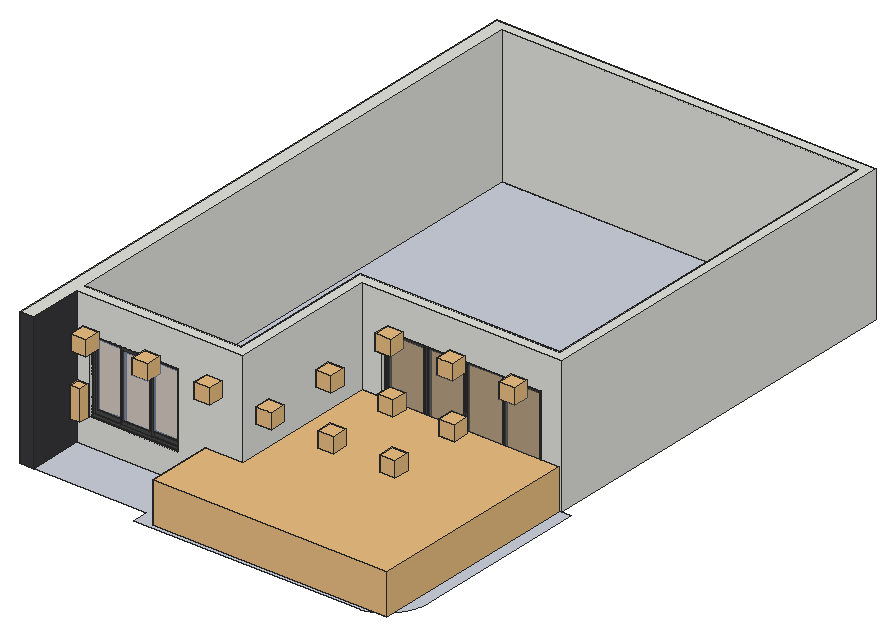
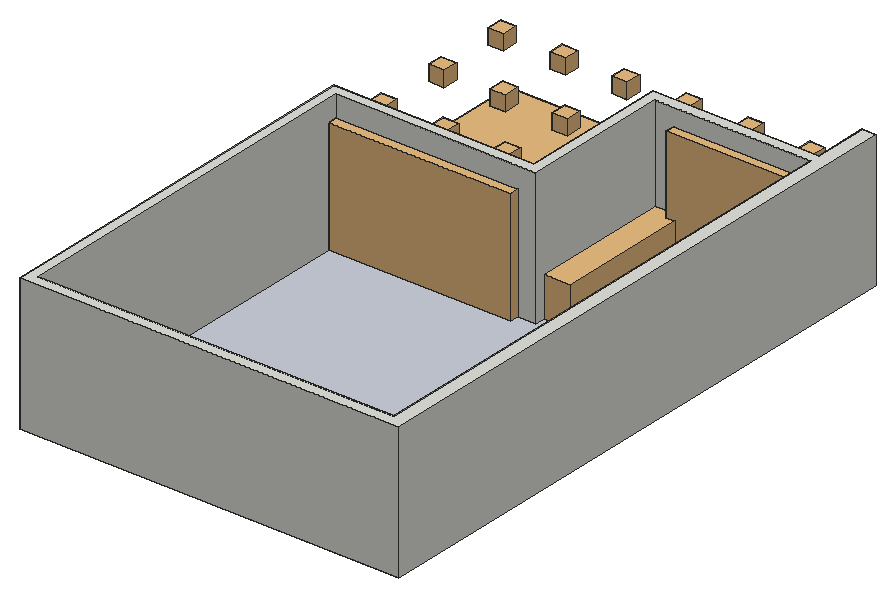
# SketchUp Ruby script. Lengths in inches.
U = 1.inch
M = Sketchup.active_model
def pt(a) = Geom::Point3d.new(a.map { |v| v * U })
def face(e, loops, mat)
  f = e.add_face(loops[0].map { |a| pt(a) })
  loops[1..].each { |l| e.add_face(l.map { |a| pt(a) }).erase! }
  f.material = f.back_material = mat if mat
  f
end
# faces: each face lists its corners as indices into pts; further lists are holes
def faces(e, pts, list, mat = nil) = list.each { |f| face(e, (f[0].is_a?(Array) ? f : [f]).map { |l| l.map { |i| pts[i] } }, mat) }
# xy, xz, yz: faces in a plane at the given z, y or x. An outline is a flat list of corners, or four numbers for a rectangle; further outlines are holes
def ring(l) = l.size == 4 ? [[l[0], l[1]], [l[2], l[1]], [l[2], l[3]], [l[0], l[3]]] : l.each_slice(2).to_a
def flat(e, list, mat, &to3) = list.each { |f| face(e, (f[0].is_a?(Array) ? f : [f]).map { |l| ring(l).map { |u, v| to3.(u, v) } }, mat) }
def xy(e, z, list, mat = nil) = flat(e, list, mat) { |x, y| [x, y, z] }
def xz(e, y, list, mat = nil) = flat(e, list, mat) { |x, z| [x, y, z] }
def yz(e, x, list, mat = nil) = flat(e, list, mat) { |y, z| [x, y, z] }
def lines(e, pts, list) = list.each { |a, b| e.add_line(pt(pts[a]), pt(pts[b])) }
# prism: a flat outline (further loops are holes) pulled along v
def prism(e, loops, v, mat = nil)
  f = face(e, loops, mat); d = Geom::Vector3d.new(v.map { |x| x * U })
  f.pushpull(f.normal.samedirection?(d) ? d.length : -d.length)
end
def box(e, o, s, mat = nil) = prism(e, [[o, [o[0] + s[0], o[1], o[2]], [o[0] + s[0], o[1] + s[1], o[2]], [o[0], o[1] + s[1], o[2]]]], [0, 0, s[2]], mat)
def at(x, y, z, deg = 0) = Geom::Transformation.translation(pt([x, y, z])) * Geom::Transformation.rotation(ORIGIN, Z_AXIS, deg.degrees)
def axes(o, x, y, z) = Geom::Transformation.new([*x, 0, *y, 0, *z, 0, *pt(o).to_a, 1])
def part(name) = M.definitions.add(name)
# library, detail: a bought-in or finely detailed component or shape, given as its bounding box
def library(name, o, s) = part(name).tap { |d| box(d.entities, o, s) }
def detail(e, o, s) = box(e.add_group.entities, o, s)
def put(e, d, t, mat = nil) = e.add_instance(d, t).tap { |i| i.material = mat if mat }
def group(e, t, mat = nil) = e.add_group.tap { |g| g.transformation = t; g.material = mat if mat }.entities
root = M.entities
M.materials.add("1432 AP 8245 TAR ROAD").color = [57, 57, 60]
M.materials.add("[Marble Carrara Floor Tile]").color = [204, 208, 219]
M.materials.add("[Steel Brushed Stainless]").color = [71, 71, 71]
M.materials.add("[Steel Brushed Stainless]1").color = [76, 76, 76]
M.materials.add("[Translucent Glass Blue]").color = [188, 212, 255]
M.materials["[Translucent Glass Blue]"].alpha = 0.5
M.materials.add("[Translucent Glass Gray]").color = [128, 128, 128]
M.materials["[Translucent Glass Gray]"].alpha = 0.5
c1 = part("Group\#13")
box(c1.entities,[0,0,0],[1.97,3.9375,10.02])
c2 = part("Group\#9")
box(c2.entities,[0,2.36,0.1],[1.97,1.58,9.67])
c3 = part("Group\#10")
xz(c3.entities,0,[[0,0,33.34,51.88]])
c4 = part("Group\#11")
xy(c4.entities,0.1,[[0,2.36,1.97,3.9375]])
xy(c4.entities,4.64,[[0.39,2.36,1.57,2.95]])
xy(c4.entities,5.23,[[0.39,2.36,1.57,2.95]])
xy(c4.entities,9.77,[[0,2.36,1.97,3.9375]])
xz(c4.entities,2.36,[[[0,0.1,1.97,9.77],[0.39,4.64,1.57,5.23]]])
xz(c4.entities,2.95,[[0.39,4.64,1.57,5.23]])
xz(c4.entities,3.9375,[[0,0.1,1.97,9.77]])
yz(c4.entities,0,[[2.36,0.1,3.9375,9.77]])
yz(c4.entities,0.39,[[2.36,4.64,2.95,5.23]])
yz(c4.entities,1.57,[[2.36,4.64,2.95,5.23]])
yz(c4.entities,1.97,[[2.36,0.1,3.9375,9.77]])
c5 = part("slide door")
p = [[0,0,0],[118.11,0,0],[0,0,80.71],[0,-3.9375,80.71],[93.24,-3.9375,80.71]]
lines(c5.entities,p,[[0,1],[2,0],[3,4]])
put(c5.entities,c1,axes([116.56,-3.9375,0],[0.78947,0,0],[0,1,0],[0,0,8.05818]))
put(c5.entities,c1,axes([0,-3.9375,0],[0.78947,0,0],[0,1,0],[0,0,8.05818]))
put(c5.entities,c1,axes([1.55,-3.9375,80.71],[0,0,-1],[0,1,0],[11.48213,0,0]))
g1 = group(c5.entities,at(1.55,-3.9375,1.97))
box(g1,[0,0,-1.97],[115,3.9375,0.79])
put(c5.entities,c2,axes([1.55,-5.91,0],[0.78947,0,0],[0,1,0],[0,0,8.05818]))
put(c5.entities,c2,axes([28.75,-5.91,0],[0.78947,0,0],[0,1,0],[0,0,8.05818]))
put(c5.entities,c2,axes([2.85,-5.91,2.76],[0,0,-1],[0,1,0],[2.65072,0,0]))
put(c5.entities,c2,axes([2.85,-5.91,78.74],[0,0,-1],[0,1,0],[2.65072,0,0]))
put(c5.entities,c3,axes([3.11,-2.76,2.76],[0.76906,0,0],[0,1,0],[0,0,1.42673]),"[Translucent Glass Gray]")
put(c5.entities,c2,axes([89.1,-5.91,78.74],[0,0,-1],[0,1,0],[2.65072,0,0]))
put(c5.entities,c3,axes([89.36,-2.76,2.76],[0.76906,0,0],[0,1,0],[0,0,1.42673]),"[Translucent Glass Gray]")
put(c5.entities,c2,axes([89.1,-5.91,2.76],[0,0,-1],[0,1,0],[2.65072,0,0]))
put(c5.entities,c2,axes([115,-5.91,0],[0.78947,0,0],[0,1,0],[0,0,8.05818]))
put(c5.entities,c2,axes([87.81,-5.91,0],[0.78947,0,0],[0,1,0],[0,0,8.05818]))
put(c5.entities,c3,axes([31.86,-1.18,2.76],[0.76906,0,0],[0,1,0],[0,0,1.42673]),"[Translucent Glass Gray]")
put(c5.entities,c2,axes([31.6,-4.33,78.74],[0,0,-1],[0,1,0],[2.65072,0,0]))
put(c5.entities,c4,axes([57.5,-4.33,0],[0.78947,0,0],[0,1,0],[0,0,8.05818]))
put(c5.entities,c2,axes([31.6,-4.33,2.76],[0,0,-1],[0,1,0],[2.65072,0,0]))
put(c5.entities,c2,axes([30.3,-4.33,0],[0.78947,0,0],[0,1,0],[0,0,8.05818]))
put(c5.entities,c2,axes([87.81,-4.33,0],[-0.78947,0,0],[0,1,0],[0,0,8.05818]))
put(c5.entities,c4,axes([60.61,-4.33,0],[-0.78947,0,0],[0,1,0],[0,0,8.05818]))
put(c5.entities,c2,axes([86.51,-4.33,2.76],[0,0,-1],[0,1,0],[-2.65072,0,0]))
put(c5.entities,c2,axes([86.51,-4.33,78.74],[0,0,-1],[0,1,0],[-2.65072,0,0]))
put(c5.entities,c3,axes([86.25,-1.18,2.76],[-0.76906,0,0],[0,1,0],[0,0,1.42673]),"[Translucent Glass Gray]")
c6 = library("Curtains",[0,0,0],[121.73,8.19,117.22])
c7 = library("Group\#23",[13.5,0,0],[216.5,192.5,50])
c8 = library("WALL LIGHT 61",[-1.86,-2.6875,-10.98],[8.43,8.43,26.69])
c9 = library("3",[-4.91,-4.91,-13.58],[13.82,13.82,13.58])
xy(root,126,[[124.5,150,324.17,150,324.66,150.09,325,150.15,325.33,150.21,325.66,150.28,325.99,150.34,326.31,150.42,326.64,150.49,327.3,150.65,327.625,150.73,327.95,150.82,328.27,150.91,328.6,151,329.24,151.2,329.5625,151.3,329.88,151.4,330.84,151.73,331.15,151.85,331.47,151.96,331.78,152.08,332.1,152.21,332.41,152.33,333.03,152.59,333.65,152.87,333.95,153.01,334.26,153.15,334.5625,153.29,334.86,153.44,335.16,153.59,335.46,153.75,335.76,153.9,336.06,154.0625,336.35,154.22,336.65,154.39,336.94,154.55,337.52,154.89,337.81,155.07,338.1,155.24,338.66,155.6,338.95,155.79,339.23,155.98,339.5,156.17,340.06,156.55,341.14,157.35,341.41,157.56,342.19,158.19,342.45,158.41,342.71,158.625,342.96,158.84,343.22,159.07,343.47,159.29,343.72,159.52,343.96,159.75,344.21,159.98,344.45,160.21,344.69,160.45,344.93,160.68,345.17,160.92,345.4,161.16,345.63,161.41,345.86,161.65,346.32,162.15,346.54,162.4,346.76,162.66,346.98,162.91,347.2,163.17,347.83,163.95,348.04,164.22,348.24,164.49,348.45,164.76,348.85,165.3,349.04,165.57,349.23,165.85,349.61,166.4,349.8,166.6875,349.98,166.97,350.16,167.25,350.52,167.83,350.6875,168.11,350.86,168.4,351.03,168.7,351.35,169.28,351.83,170.18,352.28,171.08,352.42,171.39,352.56,171.69,352.84,172.31,353.23,173.24,353.47,173.86,353.59,174.18,353.71,174.49,353.82,174.8125,353.93,175.13,354.15,175.77,354.45,176.73,354.54,177.06,354.72,177.7,354.81,178.03,354.89,178.36,354.97,178.68,355.04,179.01,355.12,179.34,355.1875,179.67,355.26,180,355.5,181.32,355.55,181.66,355.65,182.32,355.69,182.65,355.74,182.99,355.77,183.32,355.81,183.66,355.84,183.99,355.87,184.33,355.9,184.66,355.94,185.34,355.96,185.67,355.97,186.01,355.99,186.34,355.99,186.68,356,187.02,356,344,348,344,348,692,12,692,12,164,124.5,164]],"[Marble Carrara Floor Tile]")
g2 = group(root,at(24,221,126))
xy(g2,0,[[-12,-57,-12,471,324,471,324,123,306,123,306,132,315,132,315,462,0,462,0,0,138,0,138,132,165,132,165,123,147,123,147,-9,0,-9,0,-57]])
xy(g2,24,[[12,-9,90,0]])
xy(g2,90,[[12,-9,90,0],[165,123,306,132]])
xy(g2,120,[[[-12,-57,0,-57,0,-9,147,-9,147,123,324,123,324,471,-12,471],[0,0,0,462,315,462,315,132,138,132,138,0]]])
xz(g2,-57,[[-12,0,0,120]],"1432 AP 8245 TAR ROAD")
xz(g2,-9,[[[0,0,147,120],[12,24,90,90]]])
xz(g2,0,[[[0,0,138,120],[12,24,90,90]]])
xz(g2,123,[[147,0,165,0,165,90,306,90,306,0,324,0,324,120,147,120]])
xz(g2,132,[[138,0,138,120,315,120,315,0,306,0,306,90,165,90,165,0]])
xz(g2,462,[[0,0,315,120]])
xz(g2,471,[[-12,0,324,120]])
yz(g2,-12,[[-57,0,471,120]])
yz(g2,0,[[0,0,462,120]])
yz(g2,0,[[-57,0,-9,120]],"1432 AP 8245 TAR ROAD")
yz(g2,12,[[-9,24,0,90]])
yz(g2,90,[[-9,24,0,90]])
yz(g2,138,[[0,0,132,120]])
yz(g2,147,[[-9,0,123,120]])
yz(g2,165,[[123,0,132,90]])
yz(g2,306,[[123,0,132,90]])
yz(g2,315,[[132,0,462,120]])
yz(g2,324,[[123,0,471,120]])
put(g2,c5,axes([165,129.5,0],[1.1938,0,0],[0,1,0],[0,0,1.11512]),"[Steel Brushed Stainless]")
put(g2,c6,axes([154.04,132,0],[1.32227,0,0],[0,1,0],[0,0,0.864]))
put(g2,c6,axes([0,0,0],[1,0,0],[0,1,0],[0,0,0.89]))
g3 = group(g2,at(12,-7,24),"[Steel Brushed Stainless]")
xy(g3,0,[[0,0,78,3.9375]])
xy(g3,1.8,[[1.3,0,76.7,0,76.7,1.97,52.87,1.97,52.87,0.39,25.13,0.39,25.13,1.97,1.3,1.97],[25.13,0.39,27.73,1.97],[50.27,0.39,52.87,1.97],[27.3,1.97,50.7,1.97,50.7,3.54,76.7,3.54,76.7,3.9375,1.3,3.9375,1.3,3.54,27.3,3.54]])
xy(g3,4.8,[[27.3,0.39,50.7,1.18],[27.3,1.18,50.7,1.97],[3.47,1.97,25.13,2.76],[52.87,1.97,74.53,2.76],[3.47,2.76,25.13,3.54],
  [52.87,2.76,74.53,3.54]])
xy(g3,61.43,[[27.3,0.39,50.7,1.18],[27.3,1.18,50.7,1.97],[3.47,1.97,25.13,2.76],[52.87,1.97,74.53,2.76],[3.47,2.76,25.13,3.54],
  [52.87,2.76,74.53,3.54]])
xy(g3,64.2,[[1.3,0,1.3,1.97,25.13,1.97,25.13,0.39,52.87,0.39,52.87,1.97,76.7,1.97,76.7,0],[25.13,0.39,52.87,1.97],[1.3,1.97,27.3,3.54],[27.3,1.97,27.3,3.54,1.3,3.54,1.3,3.9375,76.7,3.9375,76.7,3.54,50.7,3.54,50.7,1.97]])
xy(g3,66,[[0,0,78,3.9375]])
xz(g3,0,[[[0,0,78,66],[1.3,1.8,76.7,64.2]]])
xz(g3,0.39,[[[25.13,1.8,52.87,64.2],[27.3,4.8,50.7,61.43]]])
xz(g3,1.18,[[27.3,4.8,50.7,61.43]],"[Translucent Glass Blue]")
xz(g3,1.97,[[1.3,1.8,25.13,1.8,25.13,4.8,3.47,4.8,3.47,61.43,25.13,61.43,25.13,64.2,1.3,64.2],[25.13,1.8,27.3,64.2],[27.3,1.8,50.7,4.8],[52.87,1.8,76.7,1.8,76.7,64.2,52.87,64.2,52.87,61.43,74.53,61.43,74.53,4.8,52.87,4.8],[27.3,61.43,50.7,64.2]])
xz(g3,2.76,[[3.03,61.2,3.47,62.4]])
xz(g3,2.76,[[3.47,4.8,25.13,61.43],[52.87,4.8,74.53,61.43]],"[Translucent Glass Blue]")
xz(g3,3.54,[[[1.3,1.8,27.3,64.2],[3.47,4.8,25.13,61.43]],[[50.7,1.8,76.7,64.2],[52.87,4.8,74.53,61.43]]])
xz(g3,3.9375,[[[0,0,78,66],[1.3,1.8,76.7,64.2]]])
yz(g3,0,[[0,0,3.9375,66]])
yz(g3,1.3,[[0,1.8,1.97,64.2],[3.54,1.8,3.9375,64.2]])
yz(g3,3.47,[[1.97,4.8,2.76,61.43],[2.76,4.8,3.54,61.43]])
yz(g3,25.13,[[0.39,1.8,1.97,64.2],[1.97,4.8,2.76,61.43],[2.76,4.8,3.54,61.43]])
yz(g3,27.3,[[1.97,1.8,3.54,64.2],[0.39,4.8,1.18,61.43],[1.18,4.8,1.97,61.43]])
yz(g3,50.7,[[1.97,1.8,3.54,64.2],[0.39,4.8,1.18,61.43],[1.18,4.8,1.97,61.43]])
yz(g3,52.87,[[0.39,1.8,1.97,64.2],[1.97,4.8,2.76,61.43],[2.76,4.8,3.54,61.43]])
yz(g3,74.53,[[1.97,4.8,2.76,61.43],[2.76,4.8,3.54,61.43]])
yz(g3,76.7,[[0,1.8,1.97,64.2],[3.54,1.8,3.9375,64.2]])
yz(g3,78,[[0,0,3.9375,66]])
p = [[3.03,2.76,64.2],[3.03,2.76,62.4]]
lines(g3,p,[[0,1]])
put(root,c7,axes([125.04,153.42,126],[0.96,0,0],[0,0.99,0],[0,0,0.71239]),"[Steel Brushed Stainless]1")
put(root,c8,at(64.21,159.59,193.17))
put(root,c9,at(102.8,186,232.26))
put(root,c9,at(48,186,232.26))
put(root,c9,at(212.4,186,232.26))
put(root,c9,at(157.6,186,232.26))
put(root,c9,at(212.4,252,232.26))
put(root,c9,at(212.4,318,232.26))
put(root,c9,at(322,186,232.26))
put(root,c9,at(267.2,186,232.26))
put(root,c9,at(322,252,232.26))
put(root,c9,at(267.2,252,232.26))
put(root,c9,at(322,318,232.26))
put(root,c9,at(267.2,318,232.26))
